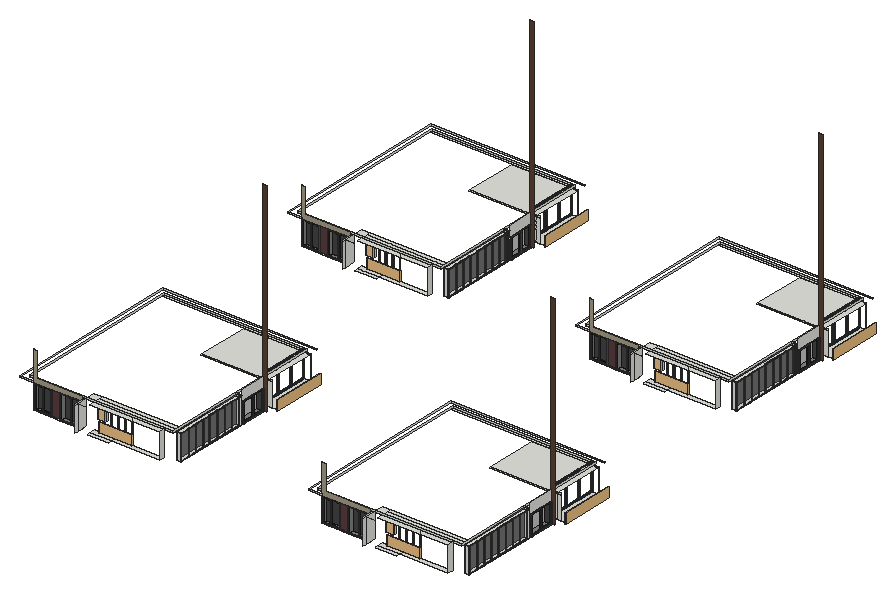
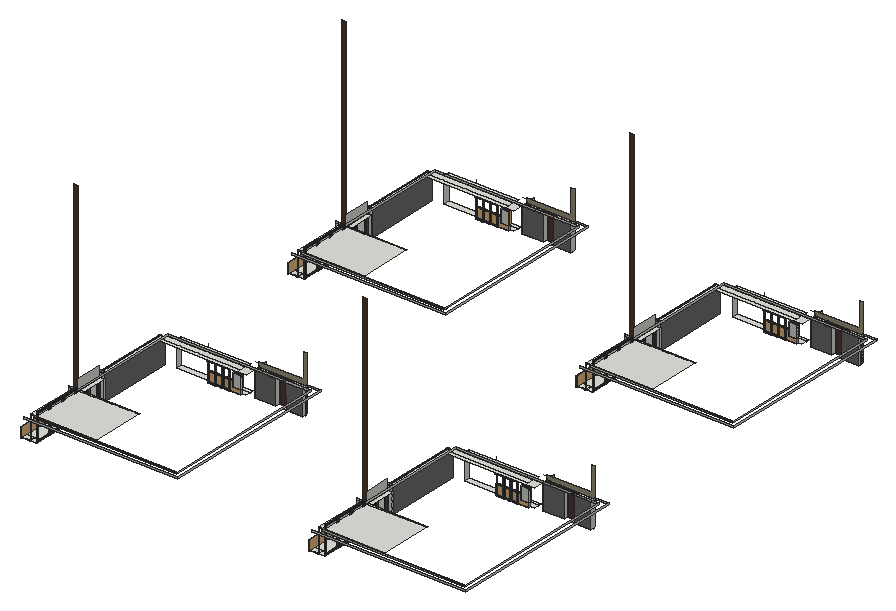
# SketchUp Ruby script. Lengths in inches.
U = 1.inch
M = Sketchup.active_model
def pt(a) = Geom::Point3d.new(a.map { |v| v * U })
def face(e, loops, mat)
  f = e.add_face(loops[0].map { |a| pt(a) })
  loops[1..].each { |l| e.add_face(l.map { |a| pt(a) }).erase! }
  f.material = f.back_material = mat if mat
  f
end
# faces: each face lists its corners as indices into pts; further lists are holes
def faces(e, pts, list, mat = nil) = list.each { |f| face(e, (f[0].is_a?(Array) ? f : [f]).map { |l| l.map { |i| pts[i] } }, mat) }
# xy, xz, yz: faces in a plane at the given z, y or x. An outline is a flat list of corners, or four numbers for a rectangle; further outlines are holes
def ring(l) = l.size == 4 ? [[l[0], l[1]], [l[2], l[1]], [l[2], l[3]], [l[0], l[3]]] : l.each_slice(2).to_a
def flat(e, list, mat, &to3) = list.each { |f| face(e, (f[0].is_a?(Array) ? f : [f]).map { |l| ring(l).map { |u, v| to3.(u, v) } }, mat) }
def xy(e, z, list, mat = nil) = flat(e, list, mat) { |x, y| [x, y, z] }
def xz(e, y, list, mat = nil) = flat(e, list, mat) { |x, z| [x, y, z] }
def yz(e, x, list, mat = nil) = flat(e, list, mat) { |y, z| [x, y, z] }
def lines(e, pts, list) = list.each { |a, b| e.add_line(pt(pts[a]), pt(pts[b])) }
# prism: a flat outline (further loops are holes) pulled along v
def prism(e, loops, v, mat = nil)
  f = face(e, loops, mat); d = Geom::Vector3d.new(v.map { |x| x * U })
  f.pushpull(f.normal.samedirection?(d) ? d.length : -d.length)
end
def box(e, o, s, mat = nil) = prism(e, [[o, [o[0] + s[0], o[1], o[2]], [o[0] + s[0], o[1] + s[1], o[2]], [o[0], o[1] + s[1], o[2]]]], [0, 0, s[2]], mat)
def at(x, y, z, deg = 0) = Geom::Transformation.translation(pt([x, y, z])) * Geom::Transformation.rotation(ORIGIN, Z_AXIS, deg.degrees)
def axes(o, x, y, z) = Geom::Transformation.new([*x, 0, *y, 0, *z, 0, *pt(o).to_a, 1])
def part(name) = M.definitions.add(name)
# library, detail: a bought-in or finely detailed component or shape, given as its bounding box
def library(name, o, s) = part(name).tap { |d| box(d.entities, o, s) }
def detail(e, o, s) = box(e.add_group.entities, o, s)
def put(e, d, t, mat = nil) = e.add_instance(d, t).tap { |i| i.material = mat if mat }
def group(e, t, mat = nil) = e.add_group.tap { |g| g.transformation = t; g.material = mat if mat }.entities
root = M.entities
M.materials.add("Glass_Tinted_Gray").color = [0, 0, 0]
M.materials["Glass_Tinted_Gray"].alpha = 0.125
M.materials.add("Glazing").color = [128, 128, 128]
M.materials["Glazing"].alpha = 0.05
M.materials.add("Powdercoating").color = [41, 44, 40]
M.materials.add("Wine2").color = [0, 0, 0]
M.materials["Wine2"].alpha = 0
M.materials.add("[0130_Gainsboro]").color = [39, 45, 50]
M.materials.add("[0135_DarkGray]").color = [81, 81, 81]
M.materials.add("[Color M05]").color = [114, 114, 114]
M.materials.add("[Color M06]").color = [86, 86, 86]
M.materials.add("[Concrete Tile]").color = [165, 155, 133]
M.materials.add("[Granite Brown]").color = [89, 59, 61]
M.materials.add("[Granite Brown]1").color = [89, 63, 50]
M.materials.add("[Mirror 02]").color = [229, 229, 229]
M.materials.add("[Terrazzo Light Blue]").color = [196, 214, 227]
c1 = library("Glass Railing",[0,0,0],[139.5,4.76,42])
c2 = part("Group\#15")
xy(c2.entities,0,[[0,-55.94,0.71,45.94]])
xy(c2.entities,0.2,[[0,-55.94,0.47,45.94],[0.47,45.94,0.71,46.42]])
xy(c2.entities,2.36,[[0.47,-55.94,0.71,46.42]])
xz(c2.entities,-55.94,[[0,0,0.71,0,0.71,2.36,0.47,2.36,0.47,0.2,0,0.2]])
xz(c2.entities,45.94,[[0,0,0.71,0.2]])
xz(c2.entities,46.42,[[0.47,0.2,0.71,2.36]])
yz(c2.entities,0,[[-55.94,0,45.94,0.2]])
yz(c2.entities,0.47,[[-55.94,0.2,46.42,2.36]])
yz(c2.entities,0.71,[[-55.94,0,45.94,0,45.94,0.2,46.42,0.2,46.42,2.36,-55.94,2.36]])
c3 = part("Group\#7")
xy(c3.entities,0,[[0,-59.09,0.71,45.94]])
xy(c3.entities,0.2,[[0,-59.09,0.47,45.94],[0.47,45.94,0.71,46.42]])
xy(c3.entities,2.36,[[0.47,-59.09,0.71,46.42]])
xz(c3.entities,-59.09,[[0,0,0.71,0,0.71,2.36,0.47,2.36,0.47,0.2,0,0.2]])
xz(c3.entities,45.94,[[0,0,0.71,0.2]])
xz(c3.entities,46.42,[[0.47,0.2,0.71,2.36]])
yz(c3.entities,0,[[-59.09,0,45.94,0.2]])
yz(c3.entities,0.47,[[-59.09,0.2,46.42,2.36]])
yz(c3.entities,0.71,[[-59.09,0,45.94,0,45.94,0.2,46.42,0.2,46.42,2.36,-59.09,2.36]])
c4 = part("Group\#16")
prism(c4.entities,[[[0.47,-56.18,0.2],[0,-56.18,0.2],[0,-56.18,0],[0.71,-56.18,0],[0.71,-56.18,2.36],[0.47,-56.18,2.36]]],[0,28.68,0])
c5 = part("Group\#10")
box(c5.entities,[-0.73,0,0],[27.99,0.55,102.05])
c6 = part("Group\#18")
xy(c6.entities,0,[[0.47,-56.18,0.47,-55.47,0,-55.47,0,-28.21,1.18,-28.21,1.18,-56.18]])
xy(c6.entities,0.2,[[0.71,-56.18,1.18,-28.21],[0,-55.47,0.47,-28.21],[0.47,-28.21,0.71,-27.74]])
xy(c6.entities,2.36,[[0.47,-56.18,0.71,-27.74]])
xz(c6.entities,-56.18,[[0.47,0,1.18,0,1.18,0.2,0.71,0.2,0.71,2.36,0.47,2.36]])
xz(c6.entities,-55.47,[[0,0,0.47,0.2]])
xz(c6.entities,-28.21,[[0,0,1.18,0.2]])
xz(c6.entities,-27.74,[[0.47,0.2,0.71,2.36]])
yz(c6.entities,0,[[-55.47,0,-28.21,0.2]])
yz(c6.entities,0.47,[[-56.18,0,-55.47,0.2],[-56.18,0.2,-27.74,2.36]])
yz(c6.entities,0.71,[[-56.18,0.2,-27.74,2.36]])
yz(c6.entities,1.18,[[-56.18,0,-28.21,0.2]])
c7 = part("Group\#34")
xy(c7.entities,0,[[-20.45,0,7.76,1.22]])
xy(c7.entities,0.06,[[-20.39,0.06,7.7,1.22]])
xy(c7.entities,0.47,[[-19.98,0,7.28,0.06]])
xy(c7.entities,101.89,[[-19.98,0,7.28,0.06]])
xy(c7.entities,102.3,[[-20.39,0.06,7.7,1.22]])
xy(c7.entities,102.36,[[-20.45,0,7.76,1.22]])
xz(c7.entities,0,[[[-20.45,0,7.76,102.36],[-19.98,0.47,7.28,101.89]]])
xz(c7.entities,0.06,[[[-20.39,0.06,7.7,102.3],[-19.98,0.47,7.28,101.89]]])
xz(c7.entities,1.22,[[[-20.45,0,7.76,102.36],[-20.39,0.06,7.7,102.3]]])
yz(c7.entities,-20.45,[[0,0,1.22,102.36]])
yz(c7.entities,-20.39,[[0.06,0.06,1.22,102.3]])
yz(c7.entities,-19.98,[[0,0.47,0.06,101.89]])
yz(c7.entities,7.28,[[0,0.47,0.06,101.89]])
yz(c7.entities,7.7,[[0.06,0.06,1.22,102.3]])
yz(c7.entities,7.76,[[0,0,1.22,102.36]])
c8 = part("Group\#6")
put(c8.entities,c2,axes([27.97,0,7.875],[1,0,0],[0,0,-1],[0,1,0]),"Powdercoating")
put(c8.entities,c3,axes([0.71,0,6.8],[-1,0,0],[0,0,-0.97687],[0,1,0]),"Powdercoating")
put(c8.entities,c4,axes([-27.5,0,-38.07],[0,0,-1],[-1,0,0],[0,1,0]),"Powdercoating")
put(c8.entities,c5,at(1.12,0.35,-38.39),"Glazing")
put(c8.entities,c6,axes([-27.5,0,63.35],[0,0,1],[-1,0,0],[0,1,0]),"Powdercoating")
put(c8.entities,c7,at(20.6875,1.0625,-38.54),"Powdercoating")
c9 = part("Sliding door assembly")
put(c9.entities,c8,at(-1.18,4.5,38.86))
g1 = group(c9.entities,at(84.74,4.5,38.86))
put(g1,c2,axes([-27.97,0,7.875],[-1,0,0],[0,0,-1],[0,1,0]),"Powdercoating")
put(g1,c3,axes([-0.71,0,6.8],[1,0,0],[0,0,-0.97687],[0,1,0]),"Powdercoating")
put(g1,c4,axes([27.5,0,-38.07],[0,0,-1],[1,0,0],[0,1,0]),"Powdercoating")
put(g1,c5,axes([-1.12,0.35,-38.39],[-1,0,0],[0,1,0],[0,0,1]),"Glazing")
put(g1,c6,axes([27.5,0,63.35],[0,0,1],[1,0,0],[0,1,0]),"Powdercoating")
put(g1,c7,axes([-20.6875,1.0625,-38.54],[-1,0,0],[0,1,0],[0,0,1]),"Powdercoating")
g2 = group(c9.entities,at(56.0625,4.5,38.86))
put(g2,c2,axes([-27.97,0,7.875],[-1,0,0],[0,0,-1],[0,1,0]),"Powdercoating")
put(g2,c4,axes([27.5,0,-38.07],[0,0,-1],[1,0,0],[0,1,0]),"Powdercoating")
put(g2,c5,axes([-1.12,0.35,-38.39],[-1,0,0],[0,1,0],[0,0,1]),"Glazing")
put(g2,c6,axes([27.5,0,63.35],[0,0,1],[1,0,0],[0,1,0]),"Powdercoating")
put(g2,c7,axes([-20.6875,1.0625,-38.54],[-1,0,0],[0,1,0],[0,0,1]),"Powdercoating")
g3 = group(g2,at(-0.71,0,6.8),"Powdercoating")
xy(g3,-45.34,[[0.47,0.2,0.71,2.36]])
xy(g3,-44.88,[[0,0,0.71,0.2]])
xy(g3,57.73,[[0,0,0.71,0,0.71,2.36,0.47,2.36,0.47,0.2,0,0.2]])
xz(g3,0,[[0,-44.88,0.71,57.73]])
xz(g3,0.2,[[0.47,-45.34,0.71,-44.88],[0,-44.88,0.47,57.73]])
xz(g3,2.36,[[0.47,-45.34,0.71,57.73]])
yz(g3,0,[[0,-44.88,0.2,57.73]])
yz(g3,0.47,[[0.2,-45.34,2.36,57.73]])
yz(g3,0.71,[[0.2,-45.34,2.36,-45.34,2.36,57.73,0,57.73,0,-44.88,0.2,-44.88]])
put(c9.entities,c8,axes([-33.94,4.5,38.86],[1.14218,0,0],[0,1,0],[0,0,1]))
c10 = part("sliding door")
put(c10.entities,c9,at(0,-4.5,-0.08))
c11 = part("PENTEK_RP Fineline 50S_Sliding_DoorCase_E1")
box(c11.entities,[0,0,0],[1.51,3.66,99.27],"[0135_DarkGray]")
c12 = part("PENTEK_RP Fineline 50S_SlidingDooe_Case_E2")
box(c12.entities,[0,0,0],[96.25,3.66,1.51],"[0135_DarkGray]")
c13 = part("pentek_RP Fineline 50S_SlidingDoor_Case")
put(c13.entities,c11,at(97.76,0,0))
put(c13.entities,c12,at(1.51,0,0))
put(c13.entities,c11,at(0,0,0))
put(c13.entities,c12,at(1.51,0,97.76))
c14 = part("PENTEK_RP Fineline 50S_SlidingDoor_GlazingBead_2")
box(c14.entities,[0,0,0],[0.56,0.59,94.39],"[0135_DarkGray]")
c15 = part("PENTEK_RP Fineline 50S_SlidingDoor_Glass")
box(c15.entities,[0,0,0],[46.58,0.16,94.39],"Glass_Tinted_Gray")
c16 = part("PENTEK_RP Fineline 50S_SlidingDoor_GlazingBead")
box(c16.entities,[0,0,0],[45.47,0.59,0.56],"[0135_DarkGray]")
c17 = part("PENTEK_RP Fineline 50S_SlidingDoor_Leaf_E1")
xy(c17.entities,0,[[0,0,0.93,1.97],[0.93,1.57,1.49,1.97]],"[0135_DarkGray]")
xy(c17.entities,96.25,[[0,0,0.93,0,0.93,1.57,1.49,1.57,1.49,1.97,0,1.97]],"[0135_DarkGray]")
xz(c17.entities,0,[[0,0,0.93,96.25]],"[0135_DarkGray]")
xz(c17.entities,1.57,[[0.93,0,1.49,95.32],[0.93,95.32,1.49,96.25]],"[0135_DarkGray]")
xz(c17.entities,1.97,[[0,0,1.49,96.25]],"[0135_DarkGray]")
yz(c17.entities,0,[[0,0,1.97,96.25]],"[0135_DarkGray]")
yz(c17.entities,0.93,[[0,0,1.57,0.93],[0,0.93,1.57,95.32],[0,95.32,1.57,96.25]],"[0135_DarkGray]")
yz(c17.entities,1.49,[[1.57,0,1.97,95.32],[1.57,95.32,1.97,96.25]],"[0135_DarkGray]")
c18 = part("PENTEK_RP Fineline 50S_SlidingDoor_Leaf_E2")
xy(c18.entities,0,[[0,0,0,1.57,0.56,1.57,0.56,1.97,46.02,1.97,46.02,1.57,46.58,1.57,46.58,0]],"[0135_DarkGray]")
xy(c18.entities,0.93,[[0,0,46.58,1.57]],"[0135_DarkGray]")
xy(c18.entities,1.49,[[0.56,1.57,46.02,1.97]],"[0135_DarkGray]")
xz(c18.entities,0,[[0,0,46.58,0.93]],"[0135_DarkGray]")
xz(c18.entities,1.57,[[0,0,0.56,0.93],[46.02,0,46.58,0.93],[0.56,0.93,46.02,1.49]],"[0135_DarkGray]")
xz(c18.entities,1.97,[[0.56,0,46.02,1.49]],"[0135_DarkGray]")
yz(c18.entities,0,[[0,0,1.57,0.93]],"[0135_DarkGray]")
yz(c18.entities,0.56,[[1.57,0,1.97,0.93],[1.57,0.93,1.97,1.49]],"[0135_DarkGray]")
yz(c18.entities,46.02,[[1.57,0,1.97,0.93],[1.57,0.93,1.97,1.49]],"[0135_DarkGray]")
yz(c18.entities,46.58,[[0,0,1.57,0.93]],"[0135_DarkGray]")
c19 = part("PENTEK_RP Fineline S_SlidingDoor_Leaf1")
put(c19.entities,c14,at(0.93,0,0.93))
put(c19.entities,c14,at(46.96,0,0.93))
put(c19.entities,c15,at(1.49,1.42,0.93))
put(c19.entities,c16,at(1.49,0,0.93))
put(c19.entities,c15,at(1.49,0.59,0.93),"[Terrazzo Light Blue]")
put(c19.entities,c17,at(0,0,0))
put(c19.entities,c17,axes([48.44,0,0],[-1,0,0],[0,1,0],[0,0,1]))
put(c19.entities,c18,axes([0.93,0,96.25],[1,0,0],[0,1,0],[0,0,-1]))
put(c19.entities,c18,at(0.93,0,0))
put(c19.entities,c16,at(1.49,0,94.77))
c20 = part("PENTEK_RP Fineline 50S_SlidingDoor_Leaf2")
put(c20.entities,c15,at(1.49,1.42,0.93))
put(c20.entities,c16,at(1.49,0,94.77))
put(c20.entities,c14,at(46.96,0,0.93))
put(c20.entities,c15,at(1.49,0.59,0.93),"[Mirror 02]")
put(c20.entities,c14,at(0.93,0,0.93))
put(c20.entities,c17,at(0,0,0))
put(c20.entities,c17,axes([48.44,0,0],[-1,0,0],[0,1,0],[0,0,1]))
put(c20.entities,c16,at(1.49,0,0.93))
put(c20.entities,c18,axes([0.93,0,96.25],[1,0,0],[0,1,0],[0,0,-1]))
put(c20.entities,c18,at(0.93,0,0))
c21 = part("PENTEK - Slimmest Steel Sliding Door / Window\#1")
put(c21.entities,c13,at(0,-1.88,-0.09))
put(c21.entities,c19,at(1.51,-2.27,1.42))
put(c21.entities,c20,at(49.32,-0.3,1.42))
c22 = part("Framed glazing panel")
xy(c22.entities,0,[[0,-0.98,43.07,0],[0,0,43.07,1.4]],"[0130_Gainsboro]")
xy(c22.entities,0.3,[[0.3,-1.43,42.77,-0.98]],"[0130_Gainsboro]")
xy(c22.entities,2.95,[[2.95,-1.43,40.12,-0.63],[2.95,-0.63,40.12,0],[2.95,0,40.12,0.64],[2.95,0.64,40.12,1.4]],"[0130_Gainsboro]")
xy(c22.entities,3.54,[[3.54,-0.63,39.53,0],[3.54,0,39.53,0.64]],"[0130_Gainsboro]")
xy(c22.entities,111.8125,[[3.54,-0.63,39.53,0],[3.54,0,39.53,0.64]],"[0130_Gainsboro]")
xy(c22.entities,112.4,[[2.95,-1.43,40.12,-0.63],[2.95,-0.63,40.12,0],[2.95,0,40.12,0.64],[2.95,0.64,40.12,1.4]],"[0130_Gainsboro]")
xy(c22.entities,115.05,[[0.3,-1.43,42.77,-0.98]],"[0130_Gainsboro]")
xy(c22.entities,115.35,[[0,-0.98,43.07,0],[0,0,43.07,1.4]],"[0130_Gainsboro]")
xz(c22.entities,-1.43,[[[0.3,0.3,42.77,115.05],[2.95,2.95,40.12,112.4]]],"[0130_Gainsboro]")
xz(c22.entities,-0.98,[[[0,0,43.07,115.35],[0.3,0.3,42.77,115.05]]],"[0130_Gainsboro]")
xz(c22.entities,-0.63,[[[2.95,2.95,40.12,112.4],[3.54,3.54,39.53,111.8125]]],"[0130_Gainsboro]")
xz(c22.entities,0,[[3.54,3.54,39.53,111.8125]],"Wine2")
xz(c22.entities,0,[[[0,0,43.07,115.35],[2.95,2.95,40.12,112.4]],[[2.95,2.95,40.12,112.4],[3.54,3.54,39.53,111.8125]]],"[0130_Gainsboro]")
xz(c22.entities,0.64,[[[2.95,2.95,40.12,112.4],[3.54,3.54,39.53,111.8125]]],"[0130_Gainsboro]")
xz(c22.entities,1.4,[[[0,0,43.07,115.35],[2.95,2.95,40.12,112.4]]],"[0130_Gainsboro]")
yz(c22.entities,0,[[-0.98,0,0,115.35],[0,0,1.4,115.35]],"[0130_Gainsboro]")
yz(c22.entities,0.3,[[-1.43,0.3,-0.98,115.05]],"[0130_Gainsboro]")
yz(c22.entities,2.95,[[-1.43,2.95,-0.63,112.4],[-0.63,2.95,0,112.4],[0,2.95,0.64,112.4],[0.64,2.95,1.4,112.4]],"[0130_Gainsboro]")
yz(c22.entities,3.54,[[-0.63,3.54,0,111.8125],[0,3.54,0.64,111.8125]],"[0130_Gainsboro]")
yz(c22.entities,39.53,[[-0.63,3.54,0,111.8125],[0,3.54,0.64,111.8125]],"[0130_Gainsboro]")
yz(c22.entities,40.12,[[-1.43,2.95,-0.63,112.4],[-0.63,2.95,0,112.4],[0,2.95,0.64,112.4],[0.64,2.95,1.4,112.4]],"[0130_Gainsboro]")
yz(c22.entities,42.77,[[-1.43,0.3,-0.98,115.05]],"[0130_Gainsboro]")
yz(c22.entities,43.07,[[-0.98,0,0,115.35],[0,0,1.4,115.35]],"[0130_Gainsboro]")
c23 = part("Glazed panel assembly")
put(c23.entities,c22,axes([90.57,1.43,0],[1.05148,0,0],[0,1,0],[0,0,1]))
put(c23.entities,c22,axes([0,1.43,0],[1.05148,0,0],[0,1,0],[0,0,1]))
put(c23.entities,c22,axes([45.29,1.43,0],[1.05148,0,0],[0,1,0],[0,0,1]))
c24 = library("Klein+raam",[128.36,12.7,0],[19.68,5.51,55.12])
xy(root,900.6875,[[557.88,1786.97,647.87,1799.9375],[1776.07,1786.97,1866.06,1799.9375],[557.88,1799.9375,647.87,1822.9375],[647.87,1799.9375,852.99,1822.9375],[1776.07,1799.9375,1866.06,1822.9375],
  [1866.06,1799.9375,2071.18,1822.9375],[894.3125,1835.1875,913.875,2148.83],[2112.5,1835.1875,2132.0625,2148.83],[557.88,3201.66,647.87,3214.625],[1776.07,3201.66,1866.06,3214.625],
  [557.88,3214.625,647.87,3237.625],[647.87,3214.625,852.99,3237.625],[1776.07,3214.625,1866.06,3237.625],[1866.06,3214.625,2071.18,3237.625],[894.3125,3249.875,913.875,3563.51],
  [2112.5,3249.875,2132.0625,3563.51]])
xy(root,900.6875,[[557.4,1786.97,557.88,1799.9375],[1775.59,1786.97,1776.07,1799.9375],[557.4,3201.66,557.88,3214.625],[1775.59,3201.66,1776.07,3214.625]],"[Granite Brown]")
xy(root,903.4375,[[319.53,1799.9375,403.0625,1822.9375],[403.0625,1799.9375,431.33,1806.5625],[431.33,1799.9375,523.04,1822.9375],[1537.72,1799.9375,1621.25,1822.9375],[1621.25,1799.9375,1649.52,1806.5625],
  [1649.52,1799.9375,1741.23,1822.9375],[319.53,3214.625,403.0625,3237.625],[403.0625,3214.625,431.33,3221.25],[431.33,3214.625,523.04,3237.625],[1537.72,3214.625,1621.25,3237.625],
  [1621.25,3214.625,1649.52,3221.25],[1649.52,3214.625,1741.23,3237.625]])
xy(root,905.36,[[890.875,2156.01,913.875,2266.33],[2109.0625,2156.01,2132.0625,2266.33],[890.875,3570.7,913.875,3681.01],[2109.0625,3570.7,2132.0625,3681.01]])
xy(root,908.8125,[[889.625,2295.875,890.875,2517.14],[890.875,2295.875,954.6875,2295.875,954.6875,2492.875,912.625,2492.875,912.625,2517.14,890.875,2517.14],[2107.8125,2295.875,2109.0625,2517.14],[2109.0625,2295.875,2172.875,2295.875,2172.875,2492.875,2130.8125,2492.875,2130.8125,2517.14,2109.0625,2517.14],[912.625,2492.875,913.875,2517.14],
  [913.875,2492.875,954.6875,2517.14],[2130.8125,2492.875,2132.0625,2517.14],[2132.0625,2492.875,2172.875,2517.14],[912.625,2517.14,913.875,2518.64],[913.875,2517.14,954.6875,2518.89],
  [2130.8125,2517.14,2132.0625,2518.64],[2132.0625,2517.14,2172.875,2518.89],[913.875,2518.89,954.6875,2520.14],[2132.0625,2518.89,2172.875,2520.14],[889.625,3710.5625,890.875,3931.82],
  [890.875,3710.5625,954.6875,3710.5625,954.6875,3907.5625,912.625,3907.5625,912.625,3931.82,890.875,3931.82],[2107.8125,3710.5625,2109.0625,3931.82],[2109.0625,3710.5625,2172.875,3710.5625,2172.875,3907.5625,2130.8125,3907.5625,2130.8125,3931.82,2109.0625,3931.82],[912.625,3907.5625,913.875,3931.82],[913.875,3907.5625,954.6875,3931.82],
  [2130.8125,3907.5625,2132.0625,3931.82],[2132.0625,3907.5625,2172.875,3931.82],[912.625,3931.82,913.875,3933.32],[913.875,3931.82,954.6875,3933.57],[2130.8125,3931.82,2132.0625,3933.32],
  [2132.0625,3931.82,2172.875,3933.57],[913.875,3933.57,954.6875,3934.82],[2132.0625,3933.57,2172.875,3934.82]])
xy(root,934.68,[[557.88,1848.875,557.88,1850.9375,557.4,1850.9375,557.4,1853.125,589.71,1853.125,589.71,1848.875],[1776.07,1848.875,1776.07,1850.9375,1775.59,1850.9375,1775.59,1853.125,1807.9,1853.125,1807.9,1848.875],[557.88,3263.5625,557.88,3265.625,557.4,3265.625,557.4,3267.8125,589.71,3267.8125,589.71,3263.5625],[1776.07,3263.5625,1776.07,3265.625,1775.59,3265.625,1775.59,3267.8125,1807.9,3267.8125,1807.9,3263.5625]])
xy(root,934.68,[[557.4,1848.875,557.88,1850.9375],[1775.59,1848.875,1776.07,1850.9375],[557.4,3263.5625,557.88,3265.625],[1775.59,3263.5625,1776.07,3265.625]],"[Granite Brown]")
xy(root,986.96,[[557.88,1848.875,589.71,1848.875,589.71,1853.125,557.4,1853.125,557.4,1850.9375,557.88,1850.9375],[1776.07,1848.875,1807.9,1848.875,1807.9,1853.125,1775.59,1853.125,1775.59,1850.9375,1776.07,1850.9375],[557.88,3263.5625,589.71,3263.5625,589.71,3267.8125,557.4,3267.8125,557.4,3265.625,557.88,3265.625],[1776.07,3263.5625,1807.9,3263.5625,1807.9,3267.8125,1775.59,3267.8125,1775.59,3265.625,1776.07,3265.625]])
xy(root,986.96,[[557.4,1848.875,557.88,1850.9375],[1775.59,1848.875,1776.07,1850.9375],[557.4,3263.5625,557.88,3265.625],[1775.59,3263.5625,1776.07,3265.625]],"[Granite Brown]")
xy(root,991.04,[[890.875,2156.01,913.875,2266.33],[2109.0625,2156.01,2132.0625,2266.33],[890.875,3570.7,913.875,3681.01],[2109.0625,3570.7,2132.0625,3681.01]])
xy(root,991.5625,[[611.65,1842.5,701.59,1850.9375],[1829.84,1842.5,1919.77,1850.9375],[611.65,3257.1875,701.59,3265.625],[1829.84,3257.1875,1919.77,3265.625]])
xy(root,1008,[[319.53,1799.9375,319.53,1822.9375,403.66,1822.9375,403.66,1806.5625,431.33,1806.5625,431.33,1822.9375,523.04,1822.9375,523.04,1799.9375],[557.88,1799.9375,852.99,1822.9375],[1537.72,1799.9375,1537.72,1822.9375,1621.85,1822.9375,1621.85,1806.5625,1649.52,1806.5625,1649.52,1822.9375,1741.23,1822.9375,1741.23,1799.9375],[1776.07,1799.9375,2071.18,1822.9375],[523.04,1822.9375,557.88,1826.625],
  [557.88,1822.9375,890.875,1826.625],[1741.23,1822.9375,1776.07,1826.625],[1776.07,1822.9375,2109.0625,1826.625],[523.04,1826.625,557.88,1826.625,557.88,1850.9375,557.4,1850.9375,557.4,1865.75,523.04,1865.75],[557.88,1826.625,890.875,1850.9375],
  [1741.23,1826.625,1776.07,1826.625,1776.07,1850.9375,1775.59,1850.9375,1775.59,1865.75,1741.23,1865.75],[1776.07,1826.625,2109.0625,1850.9375],[894.3125,1835.1875,913.875,2156.01],[2112.5,1835.1875,2132.0625,2156.01],[557.4,1850.9375,890.875,1865.75],
  [1775.59,1850.9375,2109.0625,1865.75],[635.3125,2290,890.875,2295.875],[1853.5,2290,2109.0625,2295.875],[635.3125,2295.875,890.875,2517.14],[890.875,2295.875,913.875,2517.14],
  [1853.5,2295.875,2109.0625,2517.14],[2109.0625,2295.875,2132.0625,2517.14],[890.875,2517.14,913.875,2518.64],[2109.0625,2517.14,2132.0625,2518.64],[890.875,2518.64,913.875,2518.89],
  [2109.0625,2518.64,2132.0625,2518.89],[285.875,2519.125,890.875,2531.375],[1504.0625,2519.125,2109.0625,2531.375],[319.53,3214.625,319.53,3237.625,403.66,3237.625,403.66,3221.25,431.33,3221.25,431.33,3237.625,523.04,3237.625,523.04,3214.625],[557.88,3214.625,852.99,3237.625],
  [1537.72,3214.625,1537.72,3237.625,1621.85,3237.625,1621.85,3221.25,1649.52,3221.25,1649.52,3237.625,1741.23,3237.625,1741.23,3214.625],[1776.07,3214.625,2071.18,3237.625],[523.04,3237.625,557.88,3241.3125],[557.88,3237.625,890.875,3241.3125],[1741.23,3237.625,1776.07,3241.3125],
  [1776.07,3237.625,2109.0625,3241.3125],[523.04,3241.3125,557.88,3241.3125,557.88,3265.625,557.4,3265.625,557.4,3280.4375,523.04,3280.4375],[557.88,3241.3125,890.875,3265.625],[1741.23,3241.3125,1776.07,3241.3125,1776.07,3265.625,1775.59,3265.625,1775.59,3280.4375,1741.23,3280.4375],[1776.07,3241.3125,2109.0625,3265.625],
  [894.3125,3249.875,913.875,3570.7],[2112.5,3249.875,2132.0625,3570.7],[557.4,3265.625,890.875,3280.4375],[1775.59,3265.625,2109.0625,3280.4375],[635.3125,3704.6875,890.875,3710.5625],
  [1853.5,3704.6875,2109.0625,3710.5625],[635.3125,3710.5625,890.875,3931.82],[890.875,3710.5625,913.875,3931.82],[1853.5,3710.5625,2109.0625,3931.82],[2109.0625,3710.5625,2132.0625,3931.82],
  [890.875,3931.82,913.875,3933.32],[2109.0625,3931.82,2132.0625,3933.32],[890.875,3933.32,913.875,3933.57],[2109.0625,3933.32,2132.0625,3933.57],[285.875,3933.8125,890.875,3946.0625],
  [1504.0625,3933.8125,2109.0625,3946.0625]])
xz(root,1799.9375,[[262.875,1008,319.53,1014],[1481.0625,1008,1537.72,1014]])
xz(root,1799.9375,[[319.53,1008,523.04,1008,523.04,1029.4375,334.58,1029.4375,334.58,1134,319.53,1134],[1537.72,1008,1741.23,1008,1741.23,1029.4375,1552.77,1029.4375,1552.77,1134,1537.72,1134]],"[Concrete Tile]")
xz(root,1806.5625,[[403.0625,903.4375,431.33,903.4375,431.33,1008,403.66,1008,388.85,1008.07,388.33,903.51],[1621.25,903.4375,1649.52,903.4375,1649.52,1008,1621.85,1008,1607.04,1008.07,1606.52,903.51]],"[Granite Brown]")
xz(root,1822.9375,[[285.875,1008,285.875,1014,890.875,1014,890.875,1008,403.66,1008,388.85,1008.07,388.85,1008],[388.85,1008,388.85,1008.07,403.66,1008],[1504.0625,1008,1504.0625,1014,2109.0625,1014,2109.0625,1008,1621.85,1008,1607.04,1008.07,1607.04,1008],[1607.04,1008,1607.04,1008.07,1621.85,1008]])
xz(root,1822.9375,[[319.53,903.4375,388.33,903.4375,388.85,1008,319.53,1008],[431.33,903.4375,523.04,1008],[1537.72,903.4375,1606.52,903.4375,1607.04,1008,1537.72,1008],[1649.52,903.4375,1741.23,1008]],"[Color M05]")
xz(root,1835.1875,[[894.3125,900.6875,913.875,1008],[2112.5,900.6875,2132.0625,1008]])
xz(root,1842.5,[[611.65,991.5625,701.59,993.5],[1829.84,991.5625,1919.77,993.5]])
xz(root,1848.875,[[557.88,934.68,589.71,986.96],[1776.07,934.68,1807.9,986.96]])
xz(root,1848.875,[[557.4,934.68,557.88,986.96],[1775.59,934.68,1776.07,986.96]],"[Granite Brown]")
xz(root,1853.125,[[557.4,934.68,589.71,986.96],[1775.59,934.68,1807.9,986.96]])
xz(root,2148.83,[[894.3125,900.6875,913.875,1014],[2112.5,900.6875,2132.0625,1014]])
xz(root,2156.01,[[890.875,905.36,894.3125,991.04],[894.3125,905.36,913.875,991.04],[2109.0625,905.36,2112.5,991.04],[2112.5,905.36,2132.0625,991.04],[894.3125,991.04,913.875,1008],
  [2112.5,991.04,2132.0625,1008],[894.3125,1008,913.875,1014],[2112.5,1008,2132.0625,1014]])
xz(root,2266.33,[[890.875,905.36,913.875,991.04],[2109.0625,905.36,2132.0625,991.04]],"[Color M05]")
xz(root,2266.33,[[913.875,905.36,930.75,1764],[2132.0625,905.36,2148.9375,1764]],"[Granite Brown]1")
xz(root,2295.875,[[890.875,908.8125,913.875,1008],[913.875,908.8125,930.75,1008],[2109.0625,908.8125,2132.0625,1008],[2132.0625,908.8125,2148.9375,1008],[913.875,1008,930.75,1014],
  [2132.0625,1008,2148.9375,1014]])
xz(root,2531.375,[[285.875,1008,890.875,1014],[1504.0625,1008,2109.0625,1014]])
xz(root,2554.375,[[262.875,1008,913.875,1014],[1481.0625,1008,2132.0625,1014]])
xz(root,3214.625,[[262.875,1008,319.53,1014],[1481.0625,1008,1537.72,1014]])
xz(root,3214.625,[[319.53,1008,523.04,1008,523.04,1029.4375,334.58,1029.4375,334.58,1134,319.53,1134],[1537.72,1008,1741.23,1008,1741.23,1029.4375,1552.77,1029.4375,1552.77,1134,1537.72,1134]],"[Concrete Tile]")
xz(root,3221.25,[[403.0625,903.4375,431.33,903.4375,431.33,1008,403.66,1008,388.85,1008.07,388.33,903.51],[1621.25,903.4375,1649.52,903.4375,1649.52,1008,1621.85,1008,1607.04,1008.07,1606.52,903.51]],"[Granite Brown]")
xz(root,3237.625,[[285.875,1008,285.875,1014,890.875,1014,890.875,1008,403.66,1008,388.85,1008.07,388.85,1008],[388.85,1008,388.85,1008.07,403.66,1008],[1504.0625,1008,1504.0625,1014,2109.0625,1014,2109.0625,1008,1621.85,1008,1607.04,1008.07,1607.04,1008],[1607.04,1008,1607.04,1008.07,1621.85,1008]])
xz(root,3237.625,[[319.53,903.4375,388.33,903.4375,388.85,1008,319.53,1008],[431.33,903.4375,523.04,1008],[1537.72,903.4375,1606.52,903.4375,1607.04,1008,1537.72,1008],[1649.52,903.4375,1741.23,1008]],"[Color M05]")
xz(root,3249.875,[[894.3125,900.6875,913.875,1008],[2112.5,900.6875,2132.0625,1008]])
xz(root,3257.1875,[[611.65,991.5625,701.59,993.5],[1829.84,991.5625,1919.77,993.5]])
xz(root,3263.5625,[[557.88,934.68,589.71,986.96],[1776.07,934.68,1807.9,986.96]])
xz(root,3263.5625,[[557.4,934.68,557.88,986.96],[1775.59,934.68,1776.07,986.96]],"[Granite Brown]")
xz(root,3267.8125,[[557.4,934.68,589.71,986.96],[1775.59,934.68,1807.9,986.96]])
xz(root,3563.51,[[894.3125,900.6875,913.875,1014],[2112.5,900.6875,2132.0625,1014]])
xz(root,3570.7,[[890.875,905.36,894.3125,991.04],[894.3125,905.36,913.875,991.04],[2109.0625,905.36,2112.5,991.04],[2112.5,905.36,2132.0625,991.04],[894.3125,991.04,913.875,1008],
  [2112.5,991.04,2132.0625,1008],[894.3125,1008,913.875,1014],[2112.5,1008,2132.0625,1014]])
xz(root,3681.01,[[890.875,905.36,913.875,991.04],[2109.0625,905.36,2132.0625,991.04]],"[Color M05]")
xz(root,3681.01,[[913.875,905.36,930.75,1764],[2132.0625,905.36,2148.9375,1764]],"[Granite Brown]1")
xz(root,3710.5625,[[890.875,908.8125,913.875,1008],[913.875,908.8125,930.75,1008],[2109.0625,908.8125,2132.0625,1008],[2132.0625,908.8125,2148.9375,1008],[913.875,1008,930.75,1014],
  [2132.0625,1008,2148.9375,1014]])
xz(root,3946.0625,[[285.875,1008,890.875,1014],[1504.0625,1008,2109.0625,1014]])
xz(root,3969.0625,[[262.875,1008,913.875,1014],[1481.0625,1008,2132.0625,1014]])
yz(root,262.875,[[1799.9375,1008,2554.375,1014],[3214.625,1008,3969.0625,1014]])
yz(root,285.875,[[1822.9375,1008,2531.375,1014],[3237.625,1008,3946.0625,1014]])
yz(root,319.53,[[1799.9375,903.4375,1822.9375,1008],[3214.625,903.4375,3237.625,1008]])
yz(root,431.33,[[1806.5625,903.4375,1822.9375,1008],[3221.25,903.4375,3237.625,1008]])
yz(root,523.04,[[1763.25,903.4375,1778.3125,1008],[1778.3125,903.4375,1822.9375,1008],[3177.9375,903.4375,3193,1008],[3193,903.4375,3237.625,1008],[1763.25,1008,1799.9375,1014],
  [3177.9375,1008,3214.625,1014]])
yz(root,557.4,[[1848.875,934.68,1850.9375,986.96],[1850.9375,934.68,1853.125,986.96],[3263.5625,934.68,3265.625,986.96],[3265.625,934.68,3267.8125,986.96]])
yz(root,589.71,[[1848.875,934.68,1853.125,986.96],[3263.5625,934.68,3267.8125,986.96]])
yz(root,852.99,[[1799.9375,900.6875,1822.9375,1008],[3214.625,900.6875,3237.625,1008]])
yz(root,890.875,[[1822.9375,1008,2531.375,1014],[3237.625,1008,3946.0625,1014]])
yz(root,894.3125,[[2148.83,1008,2156.01,1014],[3563.51,1008,3570.7,1014]])
yz(root,894.3125,[[1835.1875,900.6875,2148.83,1008],[3249.875,900.6875,3563.51,1008]],"[Color M05]")
yz(root,913.875,[[2518.64,908.8125,2518.89,1008],[2518.89,908.8125,2519.125,1008],[3933.32,908.8125,3933.57,1008],[3933.57,908.8125,3933.8125,1008],[2156.01,991.04,2266.33,1031.36],
  [3570.7,991.04,3681.01,1031.36],[2148.83,1008,2156.01,1014],[3563.51,1008,3570.7,1014]])
yz(root,1481.0625,[[1799.9375,1008,2554.375,1014],[3214.625,1008,3969.0625,1014]])
yz(root,1504.0625,[[1822.9375,1008,2531.375,1014],[3237.625,1008,3946.0625,1014]])
yz(root,1537.72,[[1799.9375,903.4375,1822.9375,1008],[3214.625,903.4375,3237.625,1008]])
yz(root,1649.52,[[1806.5625,903.4375,1822.9375,1008],[3221.25,903.4375,3237.625,1008]])
yz(root,1741.23,[[1763.25,903.4375,1778.3125,1008],[1778.3125,903.4375,1822.9375,1008],[3177.9375,903.4375,3193,1008],[3193,903.4375,3237.625,1008],[1763.25,1008,1799.9375,1014],
  [3177.9375,1008,3214.625,1014]])
yz(root,1775.59,[[1848.875,934.68,1850.9375,986.96],[1850.9375,934.68,1853.125,986.96],[3263.5625,934.68,3265.625,986.96],[3265.625,934.68,3267.8125,986.96]])
yz(root,1807.9,[[1848.875,934.68,1853.125,986.96],[3263.5625,934.68,3267.8125,986.96]])
yz(root,2071.18,[[1799.9375,900.6875,1822.9375,1008],[3214.625,900.6875,3237.625,1008]])
yz(root,2109.0625,[[1822.9375,1008,2531.375,1014],[3237.625,1008,3946.0625,1014]])
yz(root,2112.5,[[2148.83,1008,2156.01,1014],[3563.51,1008,3570.7,1014]])
yz(root,2112.5,[[1835.1875,900.6875,2148.83,1008],[3249.875,900.6875,3563.51,1008]],"[Color M05]")
yz(root,2132.0625,[[2518.64,908.8125,2518.89,1008],[2518.89,908.8125,2519.125,1008],[3933.32,908.8125,3933.57,1008],[3933.57,908.8125,3933.8125,1008],[2156.01,991.04,2266.33,1031.36],
  [3570.7,991.04,3681.01,1031.36],[2148.83,1008,2156.01,1014],[3563.51,1008,3570.7,1014]])
p = [[403.66,1806.5625,1008],[403.66,1822.9375,1008],[388.85,1822.9375,1008.07],[388.85,1806.5625,1008.07],[1621.85,1806.5625,1008],[1621.85,1822.9375,1008],
  [1607.04,1822.9375,1008.07],[1607.04,1806.5625,1008.07],[403.66,3221.25,1008],[403.66,3237.625,1008],[388.85,3237.625,1008.07],[388.85,3221.25,1008.07],
  [1621.85,3221.25,1008],[1621.85,3237.625,1008],[1607.04,3237.625,1008.07],[1607.04,3221.25,1008.07],[1741.23,1778.3125,1008],[1775.59,1778.3125,1008],
  [1955.15,1799.36,1024.15],[1955.15,1799.36,1008],[523.04,1778.3125,1008],[557.4,1778.3125,1008],[736.96,1799.36,1024.15],[736.96,1799.36,1008],
  [1741.23,3193,1008],[1775.59,3193,1008],[1955.15,3214.05,1024.15],[1955.15,3214.05,1008],[523.04,3193,1008],[557.4,3193,1008],
  [736.96,3214.05,1024.15],[736.96,3214.05,1008]]
faces(root,p,[[0,1,2,3],[4,5,6,7],[8,9,10,11],[12,13,14,15]])
lines(root,p,[[16,17],[18,19],[20,21],[22,23],[24,25],[26,27],[28,29],[30,31]])
put(root,c1,at(1795.95,1821.18,897.11))
put(root,c1,at(577.76,1821.18,897.11))
put(root,c1,at(1795.95,3235.86,897.11))
put(root,c1,at(577.76,3235.86,897.11))
put(root,c10,axes([2132.0625,1879.38,900.6875],[0,1.302,0],[-1,0,0],[0,0,1.03877]))
put(root,c10,axes([913.875,1879.38,900.6875],[0,1.302,0],[-1,0,0],[0,0,1.03877]))
put(root,c10,axes([2132.0625,3294.06,900.6875],[0,1.302,0],[-1,0,0],[0,0,1.03877]))
put(root,c10,axes([913.875,3294.06,900.6875],[0,1.302,0],[-1,0,0],[0,0,1.03877]))
put(root,c21,axes([1537.72,1806.83,901.03],[0.71217,0,0],[0,0.88,0],[0,0,1.054]))
put(root,c21,axes([319.53,1806.83,901.03],[0.71217,0,0],[0,0.88,0],[0,0,1.054]))
put(root,c21,axes([1537.72,3221.52,901.03],[0.71217,0,0],[0,0.88,0],[0,0,1.054]))
put(root,c21,axes([319.53,3221.52,901.03],[0.71217,0,0],[0,0.88,0],[0,0,1.054]))
put(root,c10,axes([2131,2032.98,901.42],[0,1.302,0],[-1,0,0],[0,0,1.03877]))
put(root,c10,axes([912.8125,2032.98,901.42],[0,1.302,0],[-1,0,0],[0,0,1.03877]))
put(root,c10,axes([2131,3447.67,901.42],[0,1.302,0],[-1,0,0],[0,0,1.03877]))
put(root,c10,axes([912.8125,3447.67,901.42],[0,1.302,0],[-1,0,0],[0,0,1.03877]))
put(root,c21,axes([2131.3,2158.32,902.8],[0,1.12181,0],[-2.51374,0,0],[0,0,0.87918]))
put(root,c21,axes([913.11,2158.32,902.8],[0,1.12181,0],[-2.51374,0,0],[0,0,0.87918]))
put(root,c21,axes([2131.3,3573.01,902.8],[0,1.12181,0],[-2.51374,0,0],[0,0,0.87918]))
put(root,c21,axes([913.11,3573.01,902.8],[0,1.12181,0],[-2.51374,0,0],[0,0,0.87918]))
put(root,c21,axes([1647.88,1801.9375,903.53],[0.94028,0,0],[0,0.88,0],[0,0,1.054]),"[Granite Brown]")
put(root,c21,axes([429.69,1801.9375,903.53],[0.94028,0,0],[0,0.88,0],[0,0,1.054]),"[Granite Brown]")
put(root,c21,axes([1647.88,3216.625,903.53],[0.94028,0,0],[0,0.88,0],[0,0,1.054]),"[Granite Brown]")
put(root,c21,axes([429.69,3216.625,903.53],[0.94028,0,0],[0,0.88,0],[0,0,1.054]),"[Granite Brown]")
put(root,c1,axes([2174.63,2295.6875,905.24],[0,1.6,0],[-1,0,0],[0,0,1]))
put(root,c1,axes([956.45,2295.6875,905.24],[0,1.6,0],[-1,0,0],[0,0,1]))
put(root,c1,axes([2174.63,3710.375,905.24],[0,1.6,0],[-1,0,0],[0,0,1]))
put(root,c1,axes([956.45,3710.375,905.24],[0,1.6,0],[-1,0,0],[0,0,1]))
put(root,c23,axes([1829.4375,1842.5,906.375],[0.6649,0,0],[0,0.61,0],[0,0,0.74986]),"[Color M06]")
put(root,c23,axes([611.25,1842.5,906.375],[0.6649,0,0],[0,0.61,0],[0,0,0.74986]),"[Color M06]")
put(root,c23,axes([1829.4375,3257.1875,906.375],[0.6649,0,0],[0,0.61,0],[0,0,0.74986]),"[Color M06]")
put(root,c23,axes([611.25,3257.1875,906.375],[0.6649,0,0],[0,0.61,0],[0,0,0.74986]),"[Color M06]")
put(root,c23,axes([2108.26,2307.8,908.8125],[0,1.54079,0],[-1,0,0],[0,0,1]))
put(root,c23,axes([890.08,2307.8,908.8125],[0,1.54079,0],[-1,0,0],[0,0,1]))
put(root,c23,axes([2108.26,3722.49,908.8125],[0,1.54079,0],[-1,0,0],[0,0,1]))
put(root,c23,axes([890.08,3722.49,908.8125],[0,1.54079,0],[-1,0,0],[0,0,1]))
put(root,c24,axes([1572.84,1831.5625,934.68],[1.58777,0,0],[0,0.68,0],[0,0,0.99202]))
put(root,c24,axes([354.65,1831.5625,934.68],[1.58777,0,0],[0,0.68,0],[0,0,0.99202]))
put(root,c24,axes([1572.84,3246.25,934.68],[1.58777,0,0],[0,0.68,0],[0,0,0.99202]))
put(root,c24,axes([354.65,3246.25,934.68],[1.58777,0,0],[0,0.68,0],[0,0,0.99202]))
